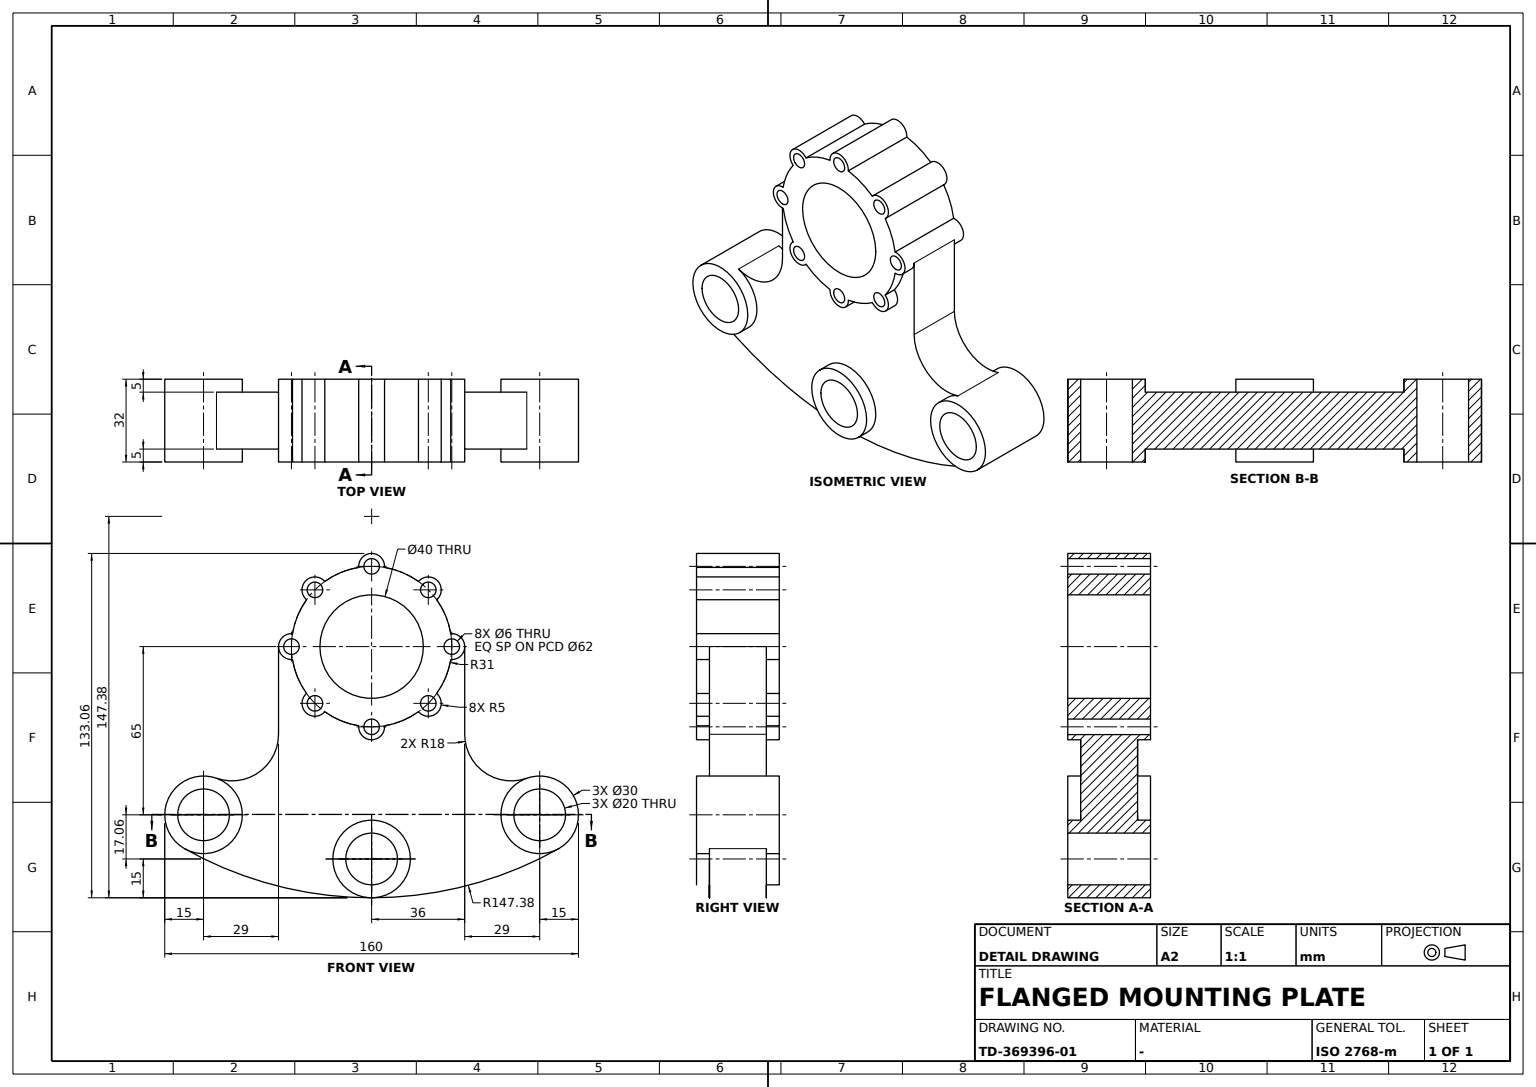
solid
v1 (16,4.9837144,30.5967742)
v2 (16,5,31)
e1 v1 v2 CIRCLE(AX(P(16,0,31),D(1,0,0),D(0,1,0)),5)
v3 (-16,4.9837144,30.5967742)
e2 v3 v1 LINE
v4 (-16,5,31)
e3 v3 v4 CIRCLE(AX(P(-16,0,31),D(1,0,0),D(0,1,0)),5)
e4 v2 v4 LINE
face CYL(AX(P(0,0,31),D(-1,0,0),D(0,1,0)),5) [-e1 -e2 e3 -e4]
v5 (-16,-15,-82.0569916)
v6 (-16,15,-82.0569916)
e5 v5 v6 CIRCLE(AX(P(-16,0,-82.0569916),D(1,0,0),D(0,1,0)),15)
e6 v6 v5 CIRCLE(AX(P(-16,0,-82.0569916),D(1,0,0),D(0,1,0)),15)
v7 (-16,10,-82.0569916)
v8 (-16,-10,-82.0569916)
e7 v7 v8 CIRCLE(AX(P(-16,0,-82.0569916),D(1,0,0),D(0,1,0)),10)
e8 v8 v7 CIRCLE(AX(P(-16,0,-82.0569916),D(1,0,0),D(0,1,0)),10)
face PLANE(AX(P(-16,0,0),D(1,0,0),D(0,1,0))) rev [-e5 -e6] [e7 e8]
v9 (11,-18.1111683,-25.1592047)
v10 (11,-4.9837144,-30.5967742)
e9 v9 v10 CIRCLE(AX(P(11,0,0),D(1,0,0),D(0,1,0)),31)
v11 (16,-4.9837144,-30.5967742)
e10 v10 v11 LINE
v12 (16,-18.1111683,-25.1592047)
e11 v12 v11 CIRCLE(AX(P(16,0,0),D(1,0,0),D(0,1,0)),31)
e12 v9 v12 LINE
face CYL(AX(P(0,0,0),D(-1,0,0),D(0,1,0)),31) [e9 e10 -e11 -e12]
v13 (16,-80,-65)
v14 (16,-50,-65)
e13 v13 v14 CIRCLE(AX(P(16,-65,-65),D(1,0,0),D(0,1,0)),15)
e14 v14 v13 CIRCLE(AX(P(16,-65,-65),D(1,0,0),D(0,1,0)),15)
v15 (16,-75,-65)
v16 (16,-55,-65)
e15 v15 v16 CIRCLE(AX(P(16,-65,-65),D(1,0,0),D(0,1,0)),10)
e16 v16 v15 CIRCLE(AX(P(16,-65,-65),D(1,0,0),D(0,1,0)),10)
face PLANE(AX(P(16,0,0),D(1,0,0),D(0,1,0))) [e13 e14] [-e15 -e16]
v17 (-11,36,0)
v18 (11,36,0)
e17 v17 v18 LINE
v19 (11,36,-33.8873016)
e18 v19 v18 LINE
v20 (-11,36,-33.8873016)
e19 v20 v19 LINE
e20 v20 v17 LINE
face PLANE(AX(P(0,36,0),D(0,-1,0),D(0,0,-1))) rev [e17 -e18 -e19 e20]
v21 (16,-25.1592047,18.1111683)
v22 (16,-30.5967742,4.9837144)
e21 v21 v22 CIRCLE(AX(P(16,0,0),D(1,0,0),D(0,1,0)),31)
v23 (-16,-25.1592047,18.1111683)
e22 v23 v21 LINE
v24 (-16,-30.5967742,4.9837144)
e23 v23 v24 CIRCLE(AX(P(-16,0,0),D(1,0,0),D(0,1,0)),31)
e24 v24 v22 LINE
face CYL(AX(P(0,0,0),D(-1,0,0),D(0,1,0)),31) [-e21 -e22 e23 e24]
v25 (-16,24.0416306,19.7989899)
v26 (-16,19.7989899,24.0416306)
e25 v25 v26 CIRCLE(AX(P(-16,21.9203102,21.9203102),D(1,0,0),D(0,0.707106781,-0.707106781)),3)
v27 (16,24.0416306,19.7989899)
e26 v27 v25 LINE
v28 (16,19.7989899,24.0416306)
e27 v27 v28 CIRCLE(AX(P(16,21.9203102,21.9203102),D(1,0,0),D(0,0.707106781,-0.707106781)),3)
e28 v28 v26 LINE
face CYL(AX(P(0,21.9203102,21.9203102),D(-1,0,0),D(0,0.707106781,-0.707106781)),3) rev [-e25 -e26 e27 e28]
v29 (-16,-24.0416306,19.7989899)
v30 (-16,-19.7989899,24.0416306)
e29 v29 v30 CIRCLE(AX(P(-16,-21.9203102,21.9203102),D(1,0,0),D(0,0.707106781,0.707106781)),3)
v31 (16,-24.0416306,19.7989899)
e30 v31 v29 LINE
v32 (16,-19.7989899,24.0416306)
e31 v31 v32 CIRCLE(AX(P(16,-21.9203102,21.9203102),D(1,0,0),D(0,0.707106781,0.707106781)),3)
e32 v32 v30 LINE
face CYL(AX(P(0,-21.9203102,21.9203102),D(-1,0,0),D(0,0.707106781,0.707106781)),3) rev [-e29 -e30 e31 e32]
v33 (-11,60,-50.8578644)
v34 (-11,50,-65)
e33 v33 v34 CIRCLE(AX(P(-11,65,-65),D(1,0,0),D(0,1,0)),15)
v35 (11,60,-50.8578644)
e34 v33 v35 LINE
v36 (11,50,-65)
e35 v35 v36 CIRCLE(AX(P(11,65,-65),D(1,0,0),D(0,1,0)),15)
v37 (16,50,-65)
e36 v36 v37 LINE
v38 (16,80,-65)
e37 v38 v37 CIRCLE(AX(P(16,65,-65),D(1,0,0),D(0,1,0)),15)
v39 (-16,80,-65)
e38 v39 v38 LINE
v40 (-16,50,-65)
e39 v39 v40 CIRCLE(AX(P(-16,65,-65),D(1,0,0),D(0,1,0)),15)
e40 v40 v34 LINE
face CYL(AX(P(0,65,-65),D(-1,0,0),D(0,1,0)),15) [-e33 e34 e35 e36 -e37 -e38 e39 e40]
v41 (16,-31,-3)
v42 (16,-31,3)
e41 v41 v42 CIRCLE(AX(P(16,-31,0),D(1,0,0),D(0,0,1)),3)
e42 v42 v41 CIRCLE(AX(P(16,-31,0),D(1,0,0),D(0,0,1)),3)
v43 (16,-5,31)
e43 v2 v43 CIRCLE(AX(P(16,0,31),D(1,0,0),D(0,1,0)),5)
v44 (16,-4.9837144,30.5967742)
e44 v43 v44 CIRCLE(AX(P(16,0,31),D(1,0,0),D(0,1,0)),5)
v45 (16,-18.1111683,25.1592047)
e45 v44 v45 CIRCLE(AX(P(16,0,0),D(1,0,0),D(0,1,0)),31)
v46 (16,-18.3847763,25.4558441)
e46 v45 v46 CIRCLE(AX(P(16,-21.9203102,21.9203102),D(1,0,0),D(0,0.707106781,0.707106781)),5)
v47 (16,-25.4558441,18.3847763)
e47 v46 v47 CIRCLE(AX(P(16,-21.9203102,21.9203102),D(1,0,0),D(0,0.707106781,0.707106781)),5)
e48 v47 v21 CIRCLE(AX(P(16,-21.9203102,21.9203102),D(1,0,0),D(0,0.707106781,0.707106781)),5)
v48 (16,-31,5)
e49 v22 v48 CIRCLE(AX(P(16,-31,0),D(1,0,0),D(0,0,1)),5)
v49 (16,-31,-5)
e50 v48 v49 CIRCLE(AX(P(16,-31,0),D(1,0,0),D(0,0,1)),5)
v50 (16,-30.5967742,-4.9837144)
e51 v49 v50 CIRCLE(AX(P(16,-31,0),D(1,0,0),D(0,0,1)),5)
v51 (16,-25.1592047,-18.1111683)
e52 v50 v51 CIRCLE(AX(P(16,0,0),D(1,0,0),D(0,1,0)),31)
v52 (16,-25.4558441,-18.3847763)
e53 v51 v52 CIRCLE(AX(P(16,-21.9203102,-21.9203102),D(1,0,0),D(0,-0.707106781,0.707106781)),5)
v53 (16,-18.3847763,-25.4558441)
e54 v52 v53 CIRCLE(AX(P(16,-21.9203102,-21.9203102),D(1,0,0),D(0,-0.707106781,0.707106781)),5)
e55 v53 v12 CIRCLE(AX(P(16,-21.9203102,-21.9203102),D(1,0,0),D(0,-0.707106781,0.707106781)),5)
v54 (16,-5,-31)
e56 v11 v54 CIRCLE(AX(P(16,0,-31),D(1,0,0),D(0,-1,0)),5)
v55 (16,5,-31)
e57 v54 v55 CIRCLE(AX(P(16,0,-31),D(1,0,0),D(0,-1,0)),5)
v56 (16,4.9837144,-30.5967742)
e58 v55 v56 CIRCLE(AX(P(16,0,-31),D(1,0,0),D(0,-1,0)),5)
v57 (16,18.1111683,-25.1592047)
e59 v56 v57 CIRCLE(AX(P(16,0,0),D(1,0,0),D(0,1,0)),31)
v58 (16,18.3847763,-25.4558441)
e60 v57 v58 CIRCLE(AX(P(16,21.9203102,-21.9203102),D(1,0,0),D(0,-0.707106781,-0.707106781)),5)
v59 (16,25.4558441,-18.3847763)
e61 v58 v59 CIRCLE(AX(P(16,21.9203102,-21.9203102),D(1,0,0),D(0,-0.707106781,-0.707106781)),5)
v60 (16,25.1592047,-18.1111683)
e62 v59 v60 CIRCLE(AX(P(16,21.9203102,-21.9203102),D(1,0,0),D(0,-0.707106781,-0.707106781)),5)
v61 (16,30.5967742,-4.9837144)
e63 v60 v61 CIRCLE(AX(P(16,0,0),D(1,0,0),D(0,1,0)),31)
v62 (16,31,-5)
e64 v61 v62 CIRCLE(AX(P(16,31,0),D(1,0,0),D(0,0,-1)),5)
v63 (16,31,5)
e65 v62 v63 CIRCLE(AX(P(16,31,0),D(1,0,0),D(0,0,-1)),5)
v64 (16,30.5967742,4.9837144)
e66 v63 v64 CIRCLE(AX(P(16,31,0),D(1,0,0),D(0,0,-1)),5)
v65 (16,25.1592047,18.1111683)
e67 v64 v65 CIRCLE(AX(P(16,0,0),D(1,0,0),D(0,1,0)),31)
v66 (16,25.4558441,18.3847763)
e68 v65 v66 CIRCLE(AX(P(16,21.9203102,21.9203102),D(1,0,0),D(0,0.707106781,-0.707106781)),5)
v67 (16,18.3847763,25.4558441)
e69 v66 v67 CIRCLE(AX(P(16,21.9203102,21.9203102),D(1,0,0),D(0,0.707106781,-0.707106781)),5)
v68 (16,18.1111683,25.1592047)
e70 v67 v68 CIRCLE(AX(P(16,21.9203102,21.9203102),D(1,0,0),D(0,0.707106781,-0.707106781)),5)
e71 v68 v1 CIRCLE(AX(P(16,0,0),D(1,0,0),D(0,1,0)),31)
v69 (16,3,-31)
v70 (16,-3,-31)
e72 v69 v70 CIRCLE(AX(P(16,0,-31),D(1,0,0),D(0,-1,0)),3)
e73 v70 v69 CIRCLE(AX(P(16,0,-31),D(1,0,0),D(0,-1,0)),3)
v71 (16,-24.0416306,-19.7989899)
v72 (16,-19.7989899,-24.0416306)
e74 v71 v72 CIRCLE(AX(P(16,-21.9203102,-21.9203102),D(1,0,0),D(0,-0.707106781,0.707106781)),3)
e75 v72 v71 CIRCLE(AX(P(16,-21.9203102,-21.9203102),D(1,0,0),D(0,-0.707106781,0.707106781)),3)
v73 (16,3,31)
v74 (16,-3,31)
e76 v73 v74 CIRCLE(AX(P(16,0,31),D(1,0,0),D(0,1,0)),3)
e77 v74 v73 CIRCLE(AX(P(16,0,31),D(1,0,0),D(0,1,0)),3)
v75 (16,31,-3)
v76 (16,31,3)
e78 v75 v76 CIRCLE(AX(P(16,31,0),D(1,0,0),D(0,0,-1)),3)
e79 v76 v75 CIRCLE(AX(P(16,31,0),D(1,0,0),D(0,0,-1)),3)
e80 v28 v27 CIRCLE(AX(P(16,21.9203102,21.9203102),D(1,0,0),D(0,0.707106781,-0.707106781)),3)
v77 (16,-20,0)
v78 (16,20,0)
e81 v77 v78 CIRCLE(AX(P(16,0,0),D(1,0,0),D(0,1,0)),20)
e82 v78 v77 CIRCLE(AX(P(16,0,0),D(1,0,0),D(0,1,0)),20)
e83 v32 v31 CIRCLE(AX(P(16,-21.9203102,21.9203102),D(1,0,0),D(0,0.707106781,0.707106781)),3)
v79 (16,24.0416306,-19.7989899)
v80 (16,19.7989899,-24.0416306)
e84 v79 v80 CIRCLE(AX(P(16,21.9203102,-21.9203102),D(1,0,0),D(0,-0.707106781,-0.707106781)),3)
e85 v80 v79 CIRCLE(AX(P(16,21.9203102,-21.9203102),D(1,0,0),D(0,-0.707106781,-0.707106781)),3)
face PLANE(AX(P(16,0,0),D(1,0,0),D(0,1,0))) [-e41 -e42] [e43 e44 e45 e46 e47 e48 e21 e49 e50 e51 e52 e53 e54 e55 e11 e56 e57 e58 e59 e60 e61 e62 e63 e64 e65 e66 e67 e68 e69 e70 e71 e1] [-e72 -e73] [-e74 -e75] [-e76 -e77] [-e78 -e79] [-e27 -e80] [-e81 -e82] [-e83 -e31] [-e84 -e85]
v81 (-11,-72.365272,-78.0672403)
v82 (11,-72.365272,-78.0672403)
e86 v81 v82 LINE
v83 (11,-50,-65)
e87 v82 v83 CIRCLE(AX(P(11,-65,-65),D(1,0,0),D(0,1,0)),15)
e88 v83 v14 LINE
v84 (-16,-80,-65)
e89 v84 v13 LINE
v85 (-16,-50,-65)
e90 v84 v85 CIRCLE(AX(P(-16,-65,-65),D(1,0,0),D(0,1,0)),15)
v86 (-11,-50,-65)
e91 v85 v86 LINE
e92 v81 v86 CIRCLE(AX(P(-11,-65,-65),D(1,0,0),D(0,1,0)),15)
face CYL(AX(P(0,-65,-65),D(-1,0,0),D(0,1,0)),15) [e86 e87 e88 -e13 -e89 e90 e91 -e92]
v87 (11,30.5967742,-4.9837144)
e93 v87 v61 LINE
v88 (11,25.1592047,-18.1111683)
e94 v88 v60 LINE
e95 v88 v87 CIRCLE(AX(P(11,0,0),D(1,0,0),D(0,1,0)),31)
face CYL(AX(P(0,0,0),D(-1,0,0),D(0,1,0)),31) [e93 -e63 -e94 e95]
v89 (-16,75,-65)
v90 (-16,55,-65)
e96 v89 v90 CIRCLE(AX(P(-16,65,-65),D(1,0,0),D(0,1,0)),10)
v91 (16,75,-65)
e97 v89 v91 LINE
v92 (16,55,-65)
e98 v91 v92 CIRCLE(AX(P(16,65,-65),D(1,0,0),D(0,1,0)),10)
e99 v90 v92 LINE
face CYL(AX(P(0,65,-65),D(-1,0,0),D(0,1,0)),10) rev [-e96 e97 e98 -e99]
e100 v26 v25 CIRCLE(AX(P(-16,21.9203102,21.9203102),D(1,0,0),D(0,0.707106781,-0.707106781)),3)
face CYL(AX(P(0,21.9203102,21.9203102),D(-1,0,0),D(0,0.707106781,-0.707106781)),3) rev [-e28 e80 e26 -e100]
v93 (-16,-75,-65)
e101 v93 v15 LINE
v94 (-16,-55,-65)
e102 v94 v16 LINE
e103 v93 v94 CIRCLE(AX(P(-16,-65,-65),D(1,0,0),D(0,1,0)),10)
face CYL(AX(P(0,-65,-65),D(-1,0,0),D(0,1,0)),10) rev [e101 e15 -e102 -e103]
v95 (-16,20,0)
v96 (-16,-20,0)
e104 v95 v96 CIRCLE(AX(P(-16,0,0),D(1,0,0),D(0,1,0)),20)
e105 v95 v78 LINE
e106 v96 v77 LINE
face CYL(AX(P(0,0,0),D(-1,0,0),D(0,1,0)),20) rev [-e104 e105 e82 -e106]
v97 (-16,-5,31)
e107 v43 v97 LINE
e108 v4 v97 CIRCLE(AX(P(-16,0,31),D(1,0,0),D(0,1,0)),5)
face CYL(AX(P(0,0,31),D(-1,0,0),D(0,1,0)),5) [-e107 -e43 e4 e108]
v98 (16,10,-82.0569916)
v99 (16,-10,-82.0569916)
e109 v98 v99 CIRCLE(AX(P(16,0,-82.0569916),D(1,0,0),D(0,1,0)),10)
e110 v99 v98 CIRCLE(AX(P(16,0,-82.0569916),D(1,0,0),D(0,1,0)),10)
v100 (16,15,-82.0569916)
v101 (16,-15,-82.0569916)
e111 v100 v101 CIRCLE(AX(P(16,0,-82.0569916),D(1,0,0),D(0,1,0)),15)
e112 v101 v100 CIRCLE(AX(P(16,0,-82.0569916),D(1,0,0),D(0,1,0)),15)
face PLANE(AX(P(16,0,0),D(1,0,0),D(0,1,0))) [-e109 -e110] [e111 e112]
v102 (-16,4.9837144,-30.5967742)
v103 (-11,4.9837144,-30.5967742)
e113 v102 v103 LINE
v104 (-16,18.1111683,-25.1592047)
e114 v102 v104 CIRCLE(AX(P(-16,0,0),D(1,0,0),D(0,1,0)),31)
v105 (-11,18.1111683,-25.1592047)
e115 v104 v105 LINE
e116 v103 v105 CIRCLE(AX(P(-11,0,0),D(1,0,0),D(0,1,0)),31)
face CYL(AX(P(0,0,0),D(-1,0,0),D(0,1,0)),31) [-e113 e114 e115 -e116]
v106 (-11,18.3847763,-25.4558441)
v107 (-11,25.4558441,-18.3847763)
e117 v106 v107 CIRCLE(AX(P(-11,21.9203102,-21.9203102),D(1,0,0),D(0,1,0)),5)
v108 (-16,18.3847763,-25.4558441)
e118 v106 v108 LINE
v109 (-16,25.4558441,-18.3847763)
e119 v108 v109 CIRCLE(AX(P(-16,21.9203102,-21.9203102),D(1,0,0),D(0,-0.707106781,-0.707106781)),5)
e120 v107 v109 LINE
face CYL(AX(P(0,21.9203102,-21.9203102),D(-1,0,0),D(0,-0.707106781,-0.707106781)),5) [-e117 e118 e119 -e120]
v110 (-16,30.5967742,-4.9837144)
v111 (-11,30.5967742,-4.9837144)
e121 v110 v111 LINE
v112 (-16,31,-5)
e122 v110 v112 CIRCLE(AX(P(-16,31,0),D(1,0,0),D(0,0,-1)),5)
v113 (-11,31,-5)
e123 v113 v112 LINE
e124 v111 v113 CIRCLE(AX(P(-11,31,0),D(1,0,0),D(0,1,0)),5)
face CYL(AX(P(0,31,0),D(-1,0,0),D(0,0,-1)),5) [-e121 e122 -e123 -e124]
v114 (-16,-4.9837144,-30.5967742)
v115 (-11,-4.9837144,-30.5967742)
e125 v114 v115 LINE
v116 (-16,-5,-31)
e126 v114 v116 CIRCLE(AX(P(-16,0,-31),D(1,0,0),D(0,-1,0)),5)
v117 (-11,-5,-31)
e127 v117 v116 LINE
e128 v115 v117 CIRCLE(AX(P(-11,0,-31),D(1,0,0),D(0,1,0)),5)
face CYL(AX(P(0,0,-31),D(-1,0,0),D(0,-1,0)),5) [-e125 e126 -e127 -e128]
v118 (-16,31,5)
e129 v63 v118 LINE
v119 (-16,30.5967742,4.9837144)
e130 v118 v119 CIRCLE(AX(P(-16,31,0),D(1,0,0),D(0,0,-1)),5)
e131 v119 v64 LINE
face CYL(AX(P(0,31,0),D(-1,0,0),D(0,0,-1)),5) [-e66 e129 e130 e131]
v120 (11,5,-31)
v121 (11,4.9837144,-30.5967742)
e132 v120 v121 CIRCLE(AX(P(11,0,-31),D(1,0,0),D(0,1,0)),5)
e133 v121 v56 LINE
e134 v55 v120 LINE
face CYL(AX(P(0,0,-31),D(-1,0,0),D(0,-1,0)),5) [e132 e133 -e58 e134]
e135 v92 v91 CIRCLE(AX(P(16,65,-65),D(1,0,0),D(0,1,0)),10)
e136 v37 v38 CIRCLE(AX(P(16,65,-65),D(1,0,0),D(0,1,0)),15)
face PLANE(AX(P(16,0,0),D(1,0,0),D(0,1,0))) [-e135 -e98] [e136 e37]
v122 (-11,72.365272,-78.0672403)
v123 (11,72.365272,-78.0672403)
e137 v122 v123 LINE
v124 (11,0,-97.0569916)
e138 v124 v123 CIRCLE(AX(P(11,0,50.3210113),D(1,0,0),D(0,1,0)),147.3780029)
e139 v82 v124 CIRCLE(AX(P(11,0,50.3210113),D(1,0,0),D(0,1,0)),147.3780029)
v125 (-11,0,-97.0569916)
e140 v81 v125 CIRCLE(AX(P(-11,0,50.3210113),D(1,0,0),D(0,1,0)),147.3780029)
e141 v125 v122 CIRCLE(AX(P(-11,0,50.3210113),D(1,0,0),D(0,1,0)),147.3780029)
face CYL(AX(P(0,0,50.3210113),D(-1,0,0),D(0,1,0)),147.3780029) [e137 -e138 -e139 -e86 e140 e141]
v126 (11,25.4558441,-18.3847763)
e142 v59 v126 LINE
e143 v126 v88 CIRCLE(AX(P(11,21.9203102,-21.9203102),D(1,0,0),D(0,1,0)),5)
face CYL(AX(P(0,21.9203102,-21.9203102),D(-1,0,0),D(0,-0.707106781,-0.707106781)),5) [e94 -e62 e142 e143]
v127 (11,-18.3847763,-25.4558441)
e144 v127 v9 CIRCLE(AX(P(11,-21.9203102,-21.9203102),D(1,0,0),D(0,1,0)),5)
v128 (11,-25.4558441,-18.3847763)
e145 v128 v127 CIRCLE(AX(P(11,-21.9203102,-21.9203102),D(1,0,0),D(0,1,0)),5)
v129 (11,-25.1592047,-18.1111683)
e146 v129 v128 CIRCLE(AX(P(11,-21.9203102,-21.9203102),D(1,0,0),D(0,1,0)),5)
v130 (11,-30.5967742,-4.9837144)
e147 v130 v129 CIRCLE(AX(P(11,0,0),D(1,0,0),D(0,1,0)),31)
v131 (11,-31,-5)
e148 v131 v130 CIRCLE(AX(P(11,-31,0),D(1,0,0),D(0,1,0)),5)
v132 (11,-36,0)
e149 v132 v131 CIRCLE(AX(P(11,-31,0),D(1,0,0),D(0,1,0)),5)
v133 (11,-36,-33.8873016)
e150 v132 v133 LINE
v134 (11,-60,-50.8578644)
e151 v133 v134 CIRCLE(AX(P(11,-54,-33.8873016),D(-1,0,0),D(0,1,0)),18)
e152 v83 v134 CIRCLE(AX(P(11,-65,-65),D(1,0,0),D(0,1,0)),15)
v135 (11,-15,-82.0569916)
e153 v135 v124 CIRCLE(AX(P(11,0,-82.0569916),D(1,0,0),D(0,1,0)),15)
v136 (11,15,-82.0569916)
e154 v136 v135 CIRCLE(AX(P(11,0,-82.0569916),D(1,0,0),D(0,1,0)),15)
e155 v124 v136 CIRCLE(AX(P(11,0,-82.0569916),D(1,0,0),D(0,1,0)),15)
e156 v36 v123 CIRCLE(AX(P(11,65,-65),D(1,0,0),D(0,1,0)),15)
e157 v35 v19 CIRCLE(AX(P(11,54,-33.8873016),D(-1,0,0),D(0,1,0)),18)
v137 (11,31,-5)
e158 v137 v18 CIRCLE(AX(P(11,31,0),D(1,0,0),D(0,1,0)),5)
e159 v87 v137 CIRCLE(AX(P(11,31,0),D(1,0,0),D(0,1,0)),5)
v138 (11,18.3847763,-25.4558441)
e160 v138 v126 CIRCLE(AX(P(11,21.9203102,-21.9203102),D(1,0,0),D(0,1,0)),5)
v139 (11,18.1111683,-25.1592047)
e161 v139 v138 CIRCLE(AX(P(11,21.9203102,-21.9203102),D(1,0,0),D(0,1,0)),5)
e162 v121 v139 CIRCLE(AX(P(11,0,0),D(1,0,0),D(0,1,0)),31)
v140 (11,-5,-31)
e163 v140 v120 CIRCLE(AX(P(11,0,-31),D(1,0,0),D(0,1,0)),5)
e164 v10 v140 CIRCLE(AX(P(11,0,-31),D(1,0,0),D(0,1,0)),5)
face PLANE(AX(P(11,0,0),D(1,0,0),D(0,1,0))) [-e144 -e145 -e146 -e147 -e148 -e149 e150 e151 -e152 -e87 e139 -e153 -e154 -e155 e138 -e156 -e35 e157 e18 -e158 -e159 -e95 -e143 -e160 -e161 -e162 -e132 -e163 -e164 -e9]
v141 (-16,-3,31)
e165 v74 v141 LINE
v142 (-16,3,31)
e166 v142 v141 CIRCLE(AX(P(-16,0,31),D(1,0,0),D(0,1,0)),3)
e167 v73 v142 LINE
face CYL(AX(P(0,0,31),D(-1,0,0),D(0,1,0)),3) rev [e165 -e166 -e167 e76]
v143 (-16,-3,-31)
e168 v70 v143 LINE
v144 (-16,3,-31)
e169 v144 v143 CIRCLE(AX(P(-16,0,-31),D(1,0,0),D(0,-1,0)),3)
e170 v69 v144 LINE
face CYL(AX(P(0,0,-31),D(-1,0,0),D(0,-1,0)),3) rev [e168 -e169 -e170 e72]
e171 v105 v106 CIRCLE(AX(P(-11,21.9203102,-21.9203102),D(1,0,0),D(0,1,0)),5)
e172 v104 v108 CIRCLE(AX(P(-16,21.9203102,-21.9203102),D(1,0,0),D(0,-0.707106781,-0.707106781)),5)
face CYL(AX(P(0,21.9203102,-21.9203102),D(-1,0,0),D(0,-0.707106781,-0.707106781)),5) [-e118 -e171 -e115 e172]
v145 (-16,-18.3847763,25.4558441)
e173 v46 v145 LINE
v146 (-16,-18.1111683,25.1592047)
e174 v146 v45 LINE
e175 v146 v145 CIRCLE(AX(P(-16,-21.9203102,21.9203102),D(1,0,0),D(0,0.707106781,0.707106781)),5)
face CYL(AX(P(0,-21.9203102,21.9203102),D(-1,0,0),D(0,0.707106781,0.707106781)),5) [-e173 -e46 -e174 e175]
v147 (-16,-4.9837144,30.5967742)
e176 v147 v44 LINE
e177 v147 v146 CIRCLE(AX(P(-16,0,0),D(1,0,0),D(0,1,0)),31)
face CYL(AX(P(0,0,0),D(-1,0,0),D(0,1,0)),31) [e174 -e45 -e176 e177]
e178 v62 v137 LINE
e179 v113 v17 CIRCLE(AX(P(-11,31,0),D(1,0,0),D(0,1,0)),5)
e180 v112 v118 CIRCLE(AX(P(-16,31,0),D(1,0,0),D(0,0,-1)),5)
face CYL(AX(P(0,31,0),D(-1,0,0),D(0,0,-1)),5) [-e129 -e65 e178 e158 -e17 -e179 e123 e180]
face CYL(AX(P(0,31,0),D(-1,0,0),D(0,0,-1)),5) [-e93 e159 -e178 -e64]
v148 (-16,-24.0416306,-19.7989899)
v149 (-16,-19.7989899,-24.0416306)
e181 v148 v149 CIRCLE(AX(P(-16,-21.9203102,-21.9203102),D(1,0,0),D(0,-0.707106781,0.707106781)),3)
e182 v149 v148 CIRCLE(AX(P(-16,-21.9203102,-21.9203102),D(1,0,0),D(0,-0.707106781,0.707106781)),3)
v150 (-16,-31,3)
v151 (-16,-31,-3)
e183 v150 v151 CIRCLE(AX(P(-16,-31,0),D(1,0,0),D(0,0,1)),3)
e184 v151 v150 CIRCLE(AX(P(-16,-31,0),D(1,0,0),D(0,0,1)),3)
e185 v96 v95 CIRCLE(AX(P(-16,0,0),D(1,0,0),D(0,1,0)),20)
e186 v143 v144 CIRCLE(AX(P(-16,0,-31),D(1,0,0),D(0,-1,0)),3)
v152 (-16,31,-3)
v153 (-16,31,3)
e187 v152 v153 CIRCLE(AX(P(-16,31,0),D(1,0,0),D(0,0,-1)),3)
e188 v153 v152 CIRCLE(AX(P(-16,31,0),D(1,0,0),D(0,0,-1)),3)
e189 v30 v29 CIRCLE(AX(P(-16,-21.9203102,21.9203102),D(1,0,0),D(0,0.707106781,0.707106781)),3)
v154 (-16,19.7989899,-24.0416306)
v155 (-16,24.0416306,-19.7989899)
e190 v154 v155 CIRCLE(AX(P(-16,21.9203102,-21.9203102),D(1,0,0),D(0,-0.707106781,-0.707106781)),3)
e191 v155 v154 CIRCLE(AX(P(-16,21.9203102,-21.9203102),D(1,0,0),D(0,-0.707106781,-0.707106781)),3)
v156 (-16,25.1592047,-18.1111683)
e192 v156 v110 CIRCLE(AX(P(-16,0,0),D(1,0,0),D(0,1,0)),31)
e193 v109 v156 CIRCLE(AX(P(-16,21.9203102,-21.9203102),D(1,0,0),D(0,-0.707106781,-0.707106781)),5)
v157 (-16,5,-31)
e194 v157 v102 CIRCLE(AX(P(-16,0,-31),D(1,0,0),D(0,-1,0)),5)
e195 v116 v157 CIRCLE(AX(P(-16,0,-31),D(1,0,0),D(0,-1,0)),5)
v158 (-16,-18.1111683,-25.1592047)
e196 v158 v114 CIRCLE(AX(P(-16,0,0),D(1,0,0),D(0,1,0)),31)
v159 (-16,-18.3847763,-25.4558441)
e197 v159 v158 CIRCLE(AX(P(-16,-21.9203102,-21.9203102),D(1,0,0),D(0,-0.707106781,0.707106781)),5)
v160 (-16,-25.4558441,-18.3847763)
e198 v160 v159 CIRCLE(AX(P(-16,-21.9203102,-21.9203102),D(1,0,0),D(0,-0.707106781,0.707106781)),5)
v161 (-16,-25.1592047,-18.1111683)
e199 v161 v160 CIRCLE(AX(P(-16,-21.9203102,-21.9203102),D(1,0,0),D(0,-0.707106781,0.707106781)),5)
v162 (-16,-30.5967742,-4.9837144)
e200 v162 v161 CIRCLE(AX(P(-16,0,0),D(1,0,0),D(0,1,0)),31)
v163 (-16,-31,-5)
e201 v163 v162 CIRCLE(AX(P(-16,-31,0),D(1,0,0),D(0,0,1)),5)
v164 (-16,-31,5)
e202 v164 v163 CIRCLE(AX(P(-16,-31,0),D(1,0,0),D(0,0,1)),5)
e203 v24 v164 CIRCLE(AX(P(-16,-31,0),D(1,0,0),D(0,0,1)),5)
v165 (-16,-25.4558441,18.3847763)
e204 v165 v23 CIRCLE(AX(P(-16,-21.9203102,21.9203102),D(1,0,0),D(0,0.707106781,0.707106781)),5)
e205 v145 v165 CIRCLE(AX(P(-16,-21.9203102,21.9203102),D(1,0,0),D(0,0.707106781,0.707106781)),5)
e206 v97 v147 CIRCLE(AX(P(-16,0,31),D(1,0,0),D(0,1,0)),5)
v166 (-16,18.1111683,25.1592047)
e207 v166 v3 CIRCLE(AX(P(-16,0,0),D(1,0,0),D(0,1,0)),31)
v167 (-16,18.3847763,25.4558441)
e208 v167 v166 CIRCLE(AX(P(-16,21.9203102,21.9203102),D(1,0,0),D(0,0.707106781,-0.707106781)),5)
v168 (-16,25.4558441,18.3847763)
e209 v168 v167 CIRCLE(AX(P(-16,21.9203102,21.9203102),D(1,0,0),D(0,0.707106781,-0.707106781)),5)
v169 (-16,25.1592047,18.1111683)
e210 v169 v168 CIRCLE(AX(P(-16,21.9203102,21.9203102),D(1,0,0),D(0,0.707106781,-0.707106781)),5)
e211 v119 v169 CIRCLE(AX(P(-16,0,0),D(1,0,0),D(0,1,0)),31)
e212 v141 v142 CIRCLE(AX(P(-16,0,31),D(1,0,0),D(0,1,0)),3)
face PLANE(AX(P(-16,0,0),D(1,0,0),D(0,1,0))) rev [e181 e182] [e183 e184] [e104 e185] [e186 e169] [e187 e188] [e29 e189] [e190 e191] [-e122 -e192 -e193 -e119 -e172 -e114 -e194 -e195 -e126 -e196 -e197 -e198 -e199 -e200 -e201 -e202 -e203 -e23 -e204 -e205 -e175 -e177 -e206 -e108 -e3 -e207 -e208 -e209 -e210 -e211 -e130 -e180] [e166 e212] [e25 e100]
e213 v71 v148 LINE
e214 v72 v149 LINE
face CYL(AX(P(0,-21.9203102,-21.9203102),D(-1,0,0),D(0,-0.707106781,0.707106781)),3) rev [-e213 e74 e214 -e181]
face CYL(AX(P(0,0,31),D(-1,0,0),D(0,1,0)),5) [-e44 e107 e206 e176]
e215 v67 v167 LINE
e216 v166 v68 LINE
face CYL(AX(P(0,21.9203102,21.9203102),D(-1,0,0),D(0,0.707106781,-0.707106781)),5) [e215 e208 e216 -e70]
e217 v130 v50 LINE
e218 v49 v131 LINE
face CYL(AX(P(0,-31,0),D(-1,0,0),D(0,0,1)),5) [e148 e217 -e51 e218]
v170 (-11,15,-82.0569916)
e219 v6 v170 LINE
e220 v125 v170 CIRCLE(AX(P(-11,0,-82.0569916),D(1,0,0),D(0,1,0)),15)
v171 (-11,-15,-82.0569916)
e221 v171 v125 CIRCLE(AX(P(-11,0,-82.0569916),D(1,0,0),D(0,1,0)),15)
e222 v5 v171 LINE
face CYL(AX(P(0,0,-82.0569916),D(-1,0,0),D(0,1,0)),15) [e219 -e220 -e221 -e222 e5]
face CYL(AX(P(0,0,31),D(-1,0,0),D(0,1,0)),3) rev [-e165 e77 e167 -e212]
e223 v90 v89 CIRCLE(AX(P(-16,65,-65),D(1,0,0),D(0,1,0)),10)
face CYL(AX(P(0,65,-65),D(-1,0,0),D(0,1,0)),10) rev [e135 -e97 -e223 e99]
e224 v94 v93 CIRCLE(AX(P(-16,-65,-65),D(1,0,0),D(0,1,0)),10)
face CYL(AX(P(0,-65,-65),D(-1,0,0),D(0,1,0)),10) rev [e102 e16 -e101 -e224]
e225 v7 v98 LINE
e226 v8 v99 LINE
face CYL(AX(P(0,0,-82.0569916),D(-1,0,0),D(0,1,0)),10) rev [e225 e109 -e226 -e7]
e227 v75 v152 LINE
e228 v76 v153 LINE
face CYL(AX(P(0,31,0),D(-1,0,0),D(0,0,-1)),3) rev [e79 e227 -e188 -e228]
e229 v33 v20 CIRCLE(AX(P(-11,54,-33.8873016),D(-1,0,0),D(0,1,0)),18)
face CYL(AX(P(0,54,-33.8873016),D(-1,0,0),D(0,1,0)),18) rev [e19 -e157 -e34 e229]
e230 v80 v154 LINE
e231 v79 v155 LINE
face CYL(AX(P(0,21.9203102,-21.9203102),D(-1,0,0),D(0,-0.707106781,-0.707106781)),3) rev [e230 -e191 -e231 e84]
e232 v53 v127 LINE
e233 v52 v128 LINE
face CYL(AX(P(0,-21.9203102,-21.9203102),D(-1,0,0),D(0,-0.707106781,0.707106781)),5) [-e232 -e54 e233 e145]
face CYL(AX(P(0,0,-31),D(-1,0,0),D(0,-1,0)),3) rev [e170 -e186 -e168 e73]
e234 v58 v138 LINE
e235 v139 v57 LINE
face CYL(AX(P(0,21.9203102,-21.9203102),D(-1,0,0),D(0,-0.707106781,-0.707106781)),5) [e161 -e234 -e60 -e235]
e236 v129 v51 LINE
face CYL(AX(P(0,0,0),D(-1,0,0),D(0,1,0)),31) [e147 e236 -e52 -e217]
e237 v48 v164 LINE
face CYL(AX(P(0,-31,0),D(-1,0,0),D(0,0,1)),5) [-e237 -e49 -e24 e203]
e238 v66 v168 LINE
face CYL(AX(P(0,21.9203102,21.9203102),D(-1,0,0),D(0,0.707106781,-0.707106781)),5) [-e69 e238 e209 -e215]
face CYL(AX(P(0,0,-82.0569916),D(-1,0,0),D(0,1,0)),10) rev [e110 -e225 -e8 e226]
e239 v54 v140 LINE
face CYL(AX(P(0,0,-31),D(-1,0,0),D(0,-1,0)),5) [-e134 -e57 e239 e163]
face CYL(AX(P(0,0,0),D(-1,0,0),D(0,1,0)),31) [-e71 -e216 e207 e2]
e240 v40 v39 CIRCLE(AX(P(-16,65,-65),D(1,0,0),D(0,1,0)),15)
face PLANE(AX(P(-16,0,0),D(1,0,0),D(0,1,0))) rev [e223 e96] [-e39 -e240]
v172 (-11,-25.4558441,-18.3847763)
e241 v172 v160 LINE
v173 (-11,-18.3847763,-25.4558441)
e242 v173 v159 LINE
e243 v172 v173 CIRCLE(AX(P(-11,-21.9203102,-21.9203102),D(1,0,0),D(0,1,0)),5)
face CYL(AX(P(0,-21.9203102,-21.9203102),D(-1,0,0),D(0,-0.707106781,0.707106781)),5) [e241 e198 -e242 -e243]
e244 v136 v100 LINE
e245 v135 v101 LINE
face CYL(AX(P(0,0,-82.0569916),D(-1,0,0),D(0,1,0)),15) [-e111 -e244 e154 e245]
v174 (-11,-31,-5)
v175 (-11,-30.5967742,-4.9837144)
e246 v174 v175 CIRCLE(AX(P(-11,-31,0),D(1,0,0),D(0,1,0)),5)
e247 v174 v163 LINE
e248 v162 v175 LINE
face CYL(AX(P(0,-31,0),D(-1,0,0),D(0,0,1)),5) [-e246 e247 e201 e248]
e249 v41 v151 LINE
e250 v42 v150 LINE
face CYL(AX(P(0,-31,0),D(-1,0,0),D(0,0,1)),3) rev [-e184 -e249 e41 e250]
v176 (-11,-18.1111683,-25.1592047)
e251 v158 v176 LINE
e252 v173 v176 CIRCLE(AX(P(-11,-21.9203102,-21.9203102),D(1,0,0),D(0,1,0)),5)
face CYL(AX(P(0,-21.9203102,-21.9203102),D(-1,0,0),D(0,-0.707106781,0.707106781)),5) [e251 -e252 e242 e197]
e253 v34 v122 CIRCLE(AX(P(-11,65,-65),D(1,0,0),D(0,1,0)),15)
face CYL(AX(P(0,65,-65),D(-1,0,0),D(0,1,0)),15) [-e36 e156 -e137 -e253 -e40 e240 e38 -e136]
face CYL(AX(P(0,31,0),D(-1,0,0),D(0,0,-1)),3) rev [e78 e228 -e187 -e227]
e254 v47 v165 LINE
face CYL(AX(P(0,-21.9203102,21.9203102),D(-1,0,0),D(0,0.707106781,0.707106781)),5) [-e48 e254 e204 e22]
v177 (-11,-25.1592047,-18.1111683)
e255 v175 v177 CIRCLE(AX(P(-11,0,0),D(1,0,0),D(0,1,0)),31)
e256 v161 v177 LINE
face CYL(AX(P(0,0,0),D(-1,0,0),D(0,1,0)),31) [-e255 -e248 e200 e256]
face CYL(AX(P(0,-21.9203102,21.9203102),D(-1,0,0),D(0,0.707106781,0.707106781)),3) rev [-e189 -e32 e83 e30]
v178 (-11,25.1592047,-18.1111683)
e257 v156 v178 LINE
e258 v107 v178 CIRCLE(AX(P(-11,21.9203102,-21.9203102),D(1,0,0),D(0,1,0)),5)
face CYL(AX(P(0,21.9203102,-21.9203102),D(-1,0,0),D(0,-0.707106781,-0.707106781)),5) [e193 e257 -e258 e120]
face CYL(AX(P(0,21.9203102,-21.9203102),D(-1,0,0),D(0,-0.707106781,-0.707106781)),5) [-e61 e234 e160 -e142]
v179 (-11,5,-31)
e259 v179 v103 CIRCLE(AX(P(-11,0,-31),D(1,0,0),D(0,1,0)),5)
e260 v179 v157 LINE
face CYL(AX(P(0,0,-31),D(-1,0,0),D(0,-1,0)),5) [-e259 e260 e194 e113]
e261 v176 v115 CIRCLE(AX(P(-11,0,0),D(1,0,0),D(0,1,0)),31)
face CYL(AX(P(0,0,0),D(-1,0,0),D(0,1,0)),31) [-e251 e196 e125 -e261]
e262 v169 v65 LINE
face CYL(AX(P(0,21.9203102,21.9203102),D(-1,0,0),D(0,0.707106781,-0.707106781)),5) [-e68 -e262 e210 -e238]
e263 v117 v179 CIRCLE(AX(P(-11,0,-31),D(1,0,0),D(0,1,0)),5)
face CYL(AX(P(0,0,-31),D(-1,0,0),D(0,-1,0)),5) [e127 e195 -e260 -e263]
face CYL(AX(P(0,0,-31),D(-1,0,0),D(0,-1,0)),5) [e164 -e239 -e56 -e10]
face CYL(AX(P(0,-21.9203102,-21.9203102),D(-1,0,0),D(0,-0.707106781,0.707106781)),5) [-e233 -e53 -e236 e146]
face CYL(AX(P(0,0,0),D(-1,0,0),D(0,1,0)),20) rev [e81 -e105 -e185 e106]
e264 v170 v171 CIRCLE(AX(P(-11,0,-82.0569916),D(1,0,0),D(0,1,0)),15)
v180 (-11,-60,-50.8578644)
e265 v86 v180 CIRCLE(AX(P(-11,-65,-65),D(1,0,0),D(0,1,0)),15)
v181 (-11,-36,-33.8873016)
e266 v181 v180 CIRCLE(AX(P(-11,-54,-33.8873016),D(-1,0,0),D(0,1,0)),18)
v182 (-11,-36,0)
e267 v182 v181 LINE
e268 v182 v174 CIRCLE(AX(P(-11,-31,0),D(1,0,0),D(0,1,0)),5)
e269 v177 v172 CIRCLE(AX(P(-11,-21.9203102,-21.9203102),D(1,0,0),D(0,1,0)),5)
e270 v178 v111 CIRCLE(AX(P(-11,0,0),D(1,0,0),D(0,1,0)),31)
face PLANE(AX(P(-11,0,0),D(1,0,0),D(0,1,0))) rev [e220 e264 e221 -e140 e92 e265 -e266 -e267 e268 e246 e255 e269 e243 e252 e261 e128 e263 e259 e116 e171 e117 e258 e270 e124 e179 -e20 -e229 e33 e253 -e141]
face CYL(AX(P(0,0,-82.0569916),D(-1,0,0),D(0,1,0)),15) [e244 -e112 -e245 e153 e155]
e271 v182 v132 LINE
face CYL(AX(P(0,-31,0),D(-1,0,0),D(0,0,1)),5) [-e268 e271 e149 -e218 -e50 e237 e202 -e247]
face CYL(AX(P(0,-21.9203102,-21.9203102),D(-1,0,0),D(0,-0.707106781,0.707106781)),5) [e232 e144 e12 -e55]
e272 v85 v84 CIRCLE(AX(P(-16,-65,-65),D(1,0,0),D(0,1,0)),15)
face PLANE(AX(P(-16,0,0),D(1,0,0),D(0,1,0))) rev [e224 e103] [-e272 -e90]
face CYL(AX(P(0,0,0),D(-1,0,0),D(0,1,0)),31) [-e133 e162 e235 -e59]
face CYL(AX(P(0,21.9203102,-21.9203102),D(-1,0,0),D(0,-0.707106781,-0.707106781)),3) rev [e85 e231 -e190 -e230]
face CYL(AX(P(0,-21.9203102,-21.9203102),D(-1,0,0),D(0,-0.707106781,0.707106781)),3) rev [e75 e213 -e182 -e214]
face CYL(AX(P(0,0,0),D(-1,0,0),D(0,1,0)),31) [-e67 -e131 e211 e262]
face CYL(AX(P(0,-31,0),D(-1,0,0),D(0,0,1)),3) rev [-e183 -e250 e42 e249]
e273 v180 v134 LINE
e274 v181 v133 LINE
face CYL(AX(P(0,-54,-33.8873016),D(-1,0,0),D(0,1,0)),18) rev [e266 e273 -e151 -e274]
face CYL(AX(P(0,0,-82.0569916),D(-1,0,0),D(0,1,0)),15) [-e264 -e219 e6 e222]
face CYL(AX(P(0,-21.9203102,21.9203102),D(-1,0,0),D(0,0.707106781,0.707106781)),5) [-e254 -e47 e173 e205]
face PLANE(AX(P(0,-36,0),D(0,1,0),D(0,0,1))) rev [e274 -e150 -e271 e267]
face CYL(AX(P(0,-65,-65),D(-1,0,0),D(0,1,0)),15) [e152 -e273 -e265 -e91 e272 e89 -e14 -e88]
face CYL(AX(P(0,0,0),D(-1,0,0),D(0,1,0)),31) [e192 e121 -e270 -e257]
face CYL(AX(P(0,-21.9203102,-21.9203102),D(-1,0,0),D(0,-0.707106781,0.707106781)),5) [-e241 -e269 -e256 e199]
